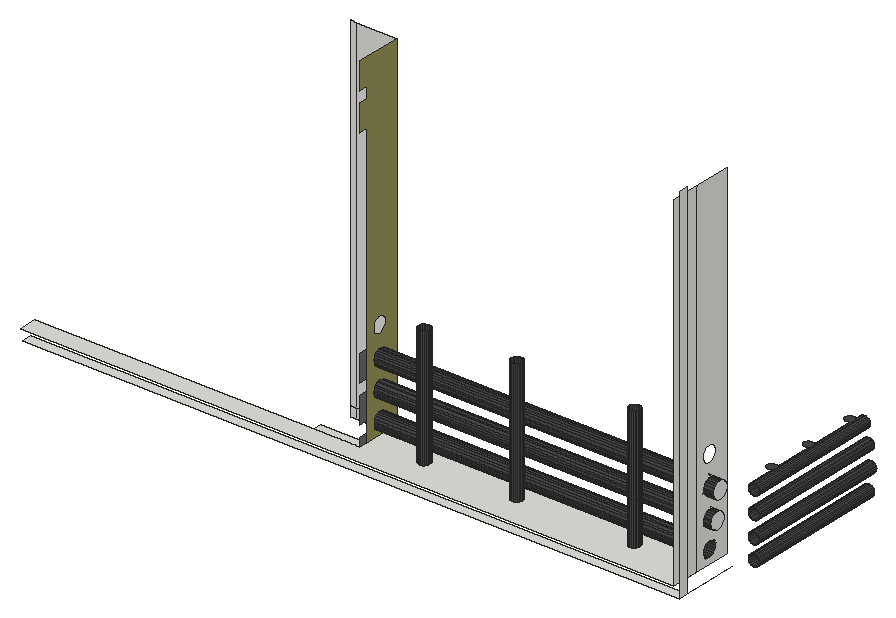
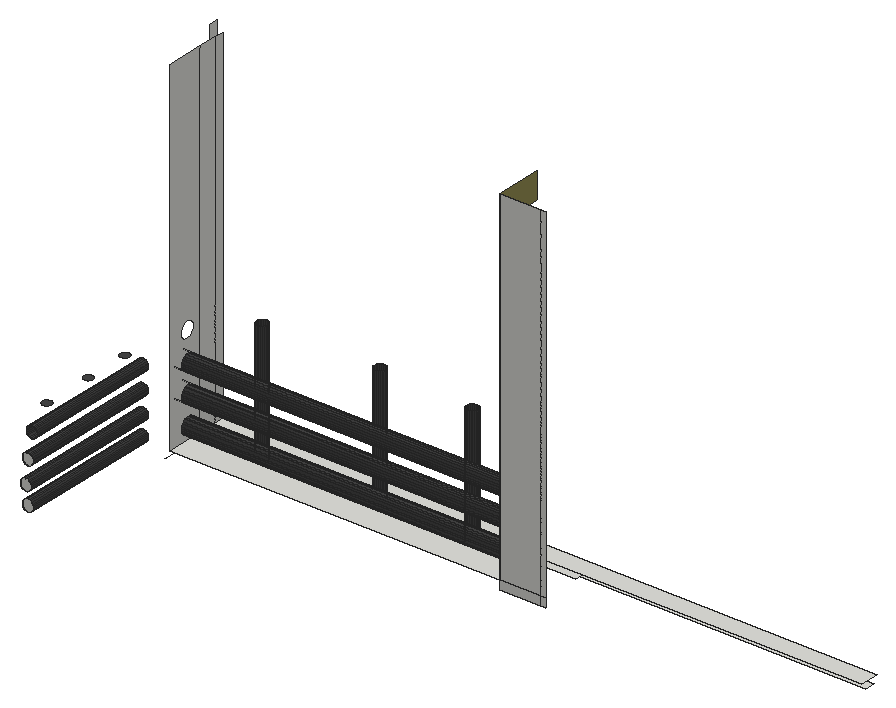
# SketchUp Ruby script. Lengths in inches.
U = 1.inch
M = Sketchup.active_model
def pt(a) = Geom::Point3d.new(a.map { |v| v * U })
def face(e, loops, mat)
  f = e.add_face(loops[0].map { |a| pt(a) })
  loops[1..].each { |l| e.add_face(l.map { |a| pt(a) }).erase! }
  f.material = f.back_material = mat if mat
  f
end
# faces: each face lists its corners as indices into pts; further lists are holes
def faces(e, pts, list, mat = nil) = list.each { |f| face(e, (f[0].is_a?(Array) ? f : [f]).map { |l| l.map { |i| pts[i] } }, mat) }
# xy, xz, yz: faces in a plane at the given z, y or x. An outline is a flat list of corners, or four numbers for a rectangle; further outlines are holes
def ring(l) = l.size == 4 ? [[l[0], l[1]], [l[2], l[1]], [l[2], l[3]], [l[0], l[3]]] : l.each_slice(2).to_a
def flat(e, list, mat, &to3) = list.each { |f| face(e, (f[0].is_a?(Array) ? f : [f]).map { |l| ring(l).map { |u, v| to3.(u, v) } }, mat) }
def xy(e, z, list, mat = nil) = flat(e, list, mat) { |x, y| [x, y, z] }
def xz(e, y, list, mat = nil) = flat(e, list, mat) { |x, z| [x, y, z] }
def yz(e, x, list, mat = nil) = flat(e, list, mat) { |y, z| [x, y, z] }
def lines(e, pts, list) = list.each { |a, b| e.add_line(pt(pts[a]), pt(pts[b])) }
# prism: a flat outline (further loops are holes) pulled along v
def prism(e, loops, v, mat = nil)
  f = face(e, loops, mat); d = Geom::Vector3d.new(v.map { |x| x * U })
  f.pushpull(f.normal.samedirection?(d) ? d.length : -d.length)
end
def box(e, o, s, mat = nil) = prism(e, [[o, [o[0] + s[0], o[1], o[2]], [o[0] + s[0], o[1] + s[1], o[2]], [o[0], o[1] + s[1], o[2]]]], [0, 0, s[2]], mat)
def at(x, y, z, deg = 0) = Geom::Transformation.translation(pt([x, y, z])) * Geom::Transformation.rotation(ORIGIN, Z_AXIS, deg.degrees)
def axes(o, x, y, z) = Geom::Transformation.new([*x, 0, *y, 0, *z, 0, *pt(o).to_a, 1])
def part(name) = M.definitions.add(name)
# library, detail: a bought-in or finely detailed component or shape, given as its bounding box
def library(name, o, s) = part(name).tap { |d| box(d.entities, o, s) }
def detail(e, o, s) = box(e.add_group.entities, o, s)
def put(e, d, t, mat = nil) = e.add_instance(d, t).tap { |i| i.material = mat if mat }
def group(e, t, mat = nil) = e.add_group.tap { |g| g.transformation = t; g.material = mat if mat }.entities
root = M.entities
M.materials.add("[0057_DarkKhaki]").color = [150, 145, 85]
M.materials.add("[0134_DimGray]").color = [105, 105, 105]
M.materials.add("[0137_Black]").color = [71, 71, 71]
xy(root,244.84,[[286.99,1.0625,497.49,4.0625]])
xy(root,247.89,[[[286.17,1.0625,495.71,1.0625,495.71,22.0625,390.0625,22.0625,390.0625,7.0625,286.17,7.0625],[437.11,9.5,436.64,9.5625,436.2,9.74,435.83,10.03,435.54,10.41,435.36,10.84,435.29,11.3125,435.36,11.78,435.54,12.22,435.83,12.6,436.2,12.88,436.64,13.0625,437.11,13.125,437.58,13.0625,438.01,12.88,438.39,12.6,438.68,12.22,438.86,11.78,438.92,11.3125,438.86,10.84,438.68,10.41,438.39,10.03,438.01,9.74,437.58,9.5625],[407.42,9.5,406.95,9.5625,406.51,9.74,406.14,10.03,405.85,10.41,405.67,10.84,405.61,11.3125,405.67,11.78,405.85,12.22,406.14,12.6,406.51,12.88,406.95,13.0625,407.42,13.125,407.89,13.0625,408.33,12.88,408.7,12.6,408.99,12.22,409.17,11.78,409.23,11.3125,409.17,10.84,408.99,10.41,408.7,10.03,408.33,9.74,407.89,9.5625],[474.86,9.5,474.39,9.5625,473.95,9.74,473.58,10.03,473.29,10.41,473.11,10.84,473.04,11.3125,473.11,11.78,473.29,12.22,473.58,12.6,473.95,12.88,474.39,13.0625,474.86,13.125,475.33,13.0625,475.76,12.88,476.14,12.6,476.43,12.22,476.61,11.78,476.67,11.3125,476.61,10.84,476.43,10.41,476.14,10.03,475.76,9.74,475.33,9.5625]],[375.29,7.0625,390.0625,10.0625]])
xy(root,274.04,[[505.89,26.06,506.26,26.11,506.6,26.25,506.9,26.48,507.13,26.78,507.27,27.125,507.32,27.5,507.27,27.87,507.13,28.22,506.9,28.51,506.6,28.74,506.26,28.89,505.89,28.93,505.51,28.89,505.17,28.74,504.87,28.51,504.64,28.22,504.5,27.87,504.45,27.5,504.5,27.125,504.64,26.78,504.87,26.48,505.17,26.25,505.51,26.11],[505.89,40.75,506.26,40.8,506.6,40.9375,506.9,41.17,507.13,41.47,507.27,41.8125,507.32,42.18,507.27,42.56,507.13,42.9,506.9,43.2,506.6,43.43,506.26,43.57,505.89,43.62,505.51,43.57,505.17,43.43,504.87,43.2,504.64,42.9,504.5,42.56,504.45,42.18,504.5,41.8125,504.64,41.47,504.87,41.17,505.17,40.9375,505.51,40.8],[505.89,57.31,506.26,57.36,506.6,57.5,506.9,57.73,507.13,58.03,507.27,58.375,507.32,58.75,507.27,59.12,507.13,59.47,506.9,59.76,506.6,59.99,506.26,60.14,505.89,60.18,505.51,60.14,505.17,59.99,504.87,59.76,504.64,59.47,504.5,59.12,504.45,58.75,504.5,58.375,504.64,58.03,504.87,57.73,505.17,57.5,505.51,57.36]],"[0137_Black]")
xz(root,22.0625,[[375.29,244.84,376.99,247.89],[376.99,244.84,390.0625,247.89],[375.29,247.89,376.99,358.6875],[376.99,247.89,390.0625,358.6875]])
xz(root,67.875,[[504.58,247.21,504.11,247.27,503.67,247.45,503.3,247.74,503.01,248.11,502.83,248.55,502.77,249.02,502.83,249.49,503.01,249.93,503.3,250.3,503.67,250.59,504.11,250.77,504.58,250.83,505.05,250.77,505.49,250.59,505.86,250.3,506.15,249.93,506.33,249.49,506.39,249.02,506.33,248.55,506.15,248.11,505.86,247.74,505.49,247.45,505.05,247.27],[504.58,260.58,504.11,260.64,503.67,260.83,503.3,261.11,503.01,261.49,502.83,261.93,502.77,262.39,502.83,262.86,503.01,263.3,503.3,263.68,503.67,263.96,504.11,264.15,504.58,264.21,505.05,264.15,505.49,263.96,505.86,263.68,506.15,263.3,506.33,262.86,506.39,262.39,506.33,261.93,506.15,261.49,505.86,261.11,505.49,260.83,505.05,260.64]])
xz(root,68.75,[[504.58,253.58,504.11,253.64,503.67,253.83,503.3,254.11,503.01,254.49,502.83,254.93,502.77,255.39,502.83,255.86,503.01,256.3,503.3,256.68,503.67,256.96,504.11,257.15,504.58,257.21,505.05,257.15,505.49,256.96,505.86,256.68,506.15,256.3,506.33,255.86,506.39,255.39,506.33,254.93,506.15,254.49,505.86,254.11,505.49,253.83,505.05,253.64]])
yz(root,390.0625,[[[10.0625,247.89,22.0625,247.89,22.0625,358.6875,7.0625,358.6875,7.0625,350.27,10.0625,350.27,10.0625,346.6875,7.0625,346.6875,7.0625,338.27,10.0625,338.27],[15.21,258.72,14.55,258.81,13.93,259.0625,13.4,259.47,12.99,260,12.73,260.62,12.65,261.28,12.73,261.95,12.99,262.5625,13.4,263.09,13.93,263.5,14.55,263.76,15.21,263.84,15.87,263.76,16.49,263.5,17.02,263.09,17.43,262.5625,17.68,261.95,17.77,261.28,17.68,260.62,17.43,260,17.02,259.47,16.49,259.0625,15.87,258.81],[15.21,267.84,14.55,267.93,13.93,268.1875,13.4,268.6,12.99,269.125,12.73,269.74,12.65,270.41,12.73,271.07,12.99,271.6875,13.4,272.22,13.93,272.625,14.55,272.88,15.21,272.97,15.87,272.88,16.49,272.625,17.02,272.22,17.43,271.6875,17.68,271.07,17.77,270.41,17.68,269.74,17.43,269.125,17.02,268.6,16.49,268.1875,15.87,267.93],[15.21,276.97,14.55,277.06,13.93,277.3125,13.4,277.72,12.99,278.25,12.73,278.87,12.65,279.53,12.73,280.2,12.99,280.8125,13.4,281.34,13.93,281.75,14.55,282.01,15.21,282.09,15.87,282.01,16.49,281.75,17.02,281.34,17.43,280.8125,17.68,280.2,17.77,279.53,17.68,278.87,17.43,278.25,17.02,277.72,16.49,277.3125,15.87,277.06],[15.21,249.59,14.55,249.68,13.93,249.9375,13.4,250.35,12.99,250.875,12.73,251.49,12.65,252.16,12.73,252.82,12.99,253.4375,13.4,253.97,13.93,254.375,14.55,254.63,15.21,254.72,15.87,254.63,16.49,254.375,17.02,253.97,17.43,253.4375,17.68,252.82,17.77,252.16,17.68,251.49,17.43,250.875,17.02,250.35,16.49,249.9375,15.87,249.68]]],"[0057_DarkKhaki]")
yz(root,390.0625,[[7.0625,247.89,10.0625,250.6875],[7.0625,254.27,10.0625,262.6875],[7.0625,266.27,10.0625,274.6875]],"[0134_DimGray]")
yz(root,495.71,[[1.0625,247.89,4.0625,358.6875],[4.0625,247.89,10.0625,358.6875],[[10.0625,247.89,22.0625,358.6875],[15.21,276.97,15.87,277.06,16.49,277.3125,17.02,277.72,17.43,278.25,17.68,278.87,17.77,279.53,17.68,280.2,17.43,280.8125,17.02,281.34,16.49,281.75,15.87,282.01,15.21,282.09,14.55,282.01,13.93,281.75,13.4,281.34,12.99,280.8125,12.73,280.2,12.65,279.53,12.73,278.87,12.99,278.25,13.4,277.72,13.93,277.3125,14.55,277.06],[15.21,249.59,15.87,249.68,16.49,249.9375,17.02,250.35,17.43,250.875,17.68,251.49,17.77,252.16,17.68,252.82,17.43,253.4375,17.02,253.97,16.49,254.375,15.87,254.63,15.21,254.72,14.55,254.63,13.93,254.375,13.4,253.97,12.99,253.4375,12.73,252.82,12.65,252.16,12.73,251.49,12.99,250.875,13.4,250.35,13.93,249.9375,14.55,249.68]]])
yz(root,497.49,[[1.0625,244.84,4.0625,361.64]])
yz(root,498.375,[[15.21,258.72,15.87,258.81,16.49,259.0625,17.02,259.47,17.43,260,17.68,260.62,17.77,261.28,17.68,261.95,17.43,262.5625,17.02,263.09,16.49,263.5,15.87,263.76,15.21,263.84,14.55,263.76,13.93,263.5,13.4,263.09,12.99,262.5625,12.73,261.95,12.65,261.28,12.73,260.62,12.99,260,13.4,259.47,13.93,259.0625,14.55,258.81]])
yz(root,499.25,[[15.21,267.84,15.87,267.93,16.49,268.1875,17.02,268.6,17.43,269.125,17.68,269.74,17.77,270.41,17.68,271.07,17.43,271.6875,17.02,272.22,16.49,272.625,15.87,272.88,15.21,272.97,14.55,272.88,13.93,272.625,13.4,272.22,12.99,271.6875,12.73,271.07,12.65,270.41,12.73,269.74,12.99,269.125,13.4,268.6,13.93,268.1875,14.55,267.93]])
p = [[504.58,22.0625,247.21],[504.11,22.0625,247.27],[504.11,67.875,247.27],[504.58,67.875,247.21],[505.05,22.0625,247.27],[505.05,67.875,247.27],
  [503.67,22.0625,247.45],[503.67,67.875,247.45],[505.49,22.0625,247.45],[505.49,67.875,247.45],[503.3,22.0625,247.74],[503.3,67.875,247.74],
  [505.86,22.0625,247.74],[505.86,67.875,247.74],[503.01,22.0625,248.11],[503.01,67.875,248.11],[506.15,22.0625,248.11],[506.15,67.875,248.11],
  [406.95,9.5625,247.89],[407.42,9.5,247.89],[407.42,9.5,286.45],[406.95,9.5625,286.45],[407.89,9.5625,247.89],[407.89,9.5625,286.45],
  [436.64,9.5625,247.89],[437.11,9.5,247.89],[437.11,9.5,287.52],[436.64,9.5625,287.52],[437.58,9.5625,247.89],[437.58,9.5625,287.52],
  [474.39,9.5625,247.89],[474.86,9.5,247.89],[474.86,9.5,287.08],[474.39,9.5625,287.08],[475.33,9.5625,247.89],[475.33,9.5625,287.08],
  [406.51,9.74,247.89],[406.51,9.74,286.45],[408.33,9.74,247.89],[408.33,9.74,286.45],[436.2,9.74,247.89],[436.2,9.74,287.52],
  [438.01,9.74,247.89],[438.01,9.74,287.52],[473.95,9.74,247.89],[473.95,9.74,287.08],[475.76,9.74,247.89],[475.76,9.74,287.08],
  [406.14,10.03,247.89],[406.14,10.03,286.45],[408.7,10.03,247.89],[408.7,10.03,286.45],[435.83,10.03,247.89],[435.83,10.03,287.52],
  [438.39,10.03,247.89],[438.39,10.03,287.52],[473.58,10.03,247.89],[473.58,10.03,287.08],[476.14,10.03,247.89],[476.14,10.03,287.08],
  [405.85,10.41,247.89],[405.85,10.41,286.45],[408.99,10.41,247.89],[408.99,10.41,286.45],[435.54,10.41,247.89],[435.54,10.41,287.52],
  [438.68,10.41,247.89],[438.68,10.41,287.52],[473.29,10.41,247.89],[473.29,10.41,287.08],[476.43,10.41,247.89],[476.43,10.41,287.08],
  [405.67,10.84,247.89],[405.67,10.84,286.45],[409.17,10.84,247.89],[409.17,10.84,286.45],[435.36,10.84,247.89],[435.36,10.84,287.52],
  [438.86,10.84,247.89],[438.86,10.84,287.52],[473.11,10.84,247.89],[473.11,10.84,287.08],[476.61,10.84,247.89],[476.61,10.84,287.08],
  [405.61,11.3125,247.89],[405.61,11.3125,286.45],[409.23,11.3125,247.89],[409.23,11.3125,286.45],[435.29,11.3125,247.89],[435.29,11.3125,287.52],
  [438.92,11.3125,247.89],[438.92,11.3125,287.52],[473.04,11.3125,247.89],[473.04,11.3125,287.08],[476.67,11.3125,247.89],[476.67,11.3125,287.08],
  [405.67,11.78,247.89],[405.67,11.78,286.45],[409.17,11.78,247.89],[409.17,11.78,286.45],[435.36,11.78,247.89],[435.36,11.78,287.52],
  [438.86,11.78,247.89],[438.86,11.78,287.52],[473.11,11.78,247.89],[473.11,11.78,287.08],[476.61,11.78,247.89],[476.61,11.78,287.08],
  [405.85,12.22,247.89],[405.85,12.22,286.45],[408.99,12.22,247.89],[408.99,12.22,286.45],[435.54,12.22,247.89],[435.54,12.22,287.52],
  [438.68,12.22,247.89],[438.68,12.22,287.52],[473.29,12.22,247.89],[473.29,12.22,287.08],[476.43,12.22,247.89],[476.43,12.22,287.08],
  [406.14,12.6,247.89],[406.14,12.6,286.45],[408.7,12.6,247.89],[408.7,12.6,286.45],[435.83,12.6,247.89],[435.83,12.6,287.52],
  [438.39,12.6,247.89],[438.39,12.6,287.52],[473.58,12.6,247.89],[473.58,12.6,287.08],[476.14,12.6,247.89],[476.14,12.6,287.08],
  [406.51,12.88,247.89],[406.51,12.88,286.45],[408.33,12.88,247.89],[408.33,12.88,286.45],[436.2,12.88,247.89],[436.2,12.88,287.52],
  [438.01,12.88,247.89],[438.01,12.88,287.52],[473.95,12.88,247.89],[473.95,12.88,287.08],[475.76,12.88,247.89],[475.76,12.88,287.08],
  [406.95,13.0625,247.89],[406.95,13.0625,286.45],[407.89,13.0625,247.89],[407.89,13.0625,286.45],[436.64,13.0625,247.89],[436.64,13.0625,287.52],
  [437.58,13.0625,247.89],[437.58,13.0625,287.52],[474.39,13.0625,247.89],[474.39,13.0625,287.08],[475.33,13.0625,247.89],[475.33,13.0625,287.08],
  [407.42,13.125,247.89],[407.42,13.125,286.45],[437.11,13.125,247.89],[437.11,13.125,287.52],[474.86,13.125,247.89],[474.86,13.125,287.08],
  [502.83,22.0625,248.55],[502.83,67.875,248.55],[506.33,22.0625,248.55],[506.33,67.875,248.55],[502.77,22.0625,249.02],[502.77,67.875,249.02],
  [506.39,22.0625,249.02],[506.39,67.875,249.02],[502.83,22.0625,249.49],[502.83,67.875,249.49],[506.33,22.0625,249.49],[506.33,67.875,249.49],
  [503.01,22.0625,249.93],[503.01,67.875,249.93],[506.15,22.0625,249.93],[506.15,67.875,249.93],[390.0625,14.55,249.68],[390.0625,15.21,249.59],
  [495.71,15.21,249.59],[495.71,14.55,249.68],[390.0625,15.87,249.68],[495.71,15.87,249.68],[390.0625,13.93,249.9375],[495.71,13.93,249.9375],
  [390.0625,16.49,249.9375],[495.71,16.49,249.9375],[390.0625,13.4,250.35],[495.71,13.4,250.35],[390.0625,17.02,250.35],[495.71,17.02,250.35],
  [503.3,22.0625,250.3],[503.3,67.875,250.3],[505.86,22.0625,250.3],[505.86,67.875,250.3],[390.0625,12.99,250.875],[495.71,12.99,250.875],
  [390.0625,17.43,250.875],[495.71,17.43,250.875],[503.67,22.0625,250.59],[503.67,67.875,250.59],[505.49,22.0625,250.59],[505.49,67.875,250.59],
  [504.11,22.0625,250.77],[504.11,67.875,250.77],[505.05,22.0625,250.77],[505.05,67.875,250.77],[504.58,22.0625,250.83],[504.58,67.875,250.83],
  [390.0625,12.73,251.49],[495.71,12.73,251.49],[390.0625,17.68,251.49],[495.71,17.68,251.49],[390.0625,12.65,252.16],[495.71,12.65,252.16],
  [390.0625,17.77,252.16],[495.71,17.77,252.16],[390.0625,12.73,252.82],[495.71,12.73,252.82],[390.0625,17.68,252.82],[495.71,17.68,252.82],
  [390.0625,12.99,253.4375],[495.71,12.99,253.4375],[390.0625,17.43,253.4375],[495.71,17.43,253.4375],[390.0625,13.4,253.97],[495.71,13.4,253.97],
  [390.0625,17.02,253.97],[495.71,17.02,253.97],[504.11,22.0625,253.64],[503.67,22.0625,253.83],[503.67,68.75,253.83],[504.11,68.75,253.64],
  [504.58,22.0625,253.58],[504.58,68.75,253.58],[505.05,22.0625,253.64],[505.05,68.75,253.64],[505.49,22.0625,253.83],[505.49,68.75,253.83],
  [503.3,22.0625,254.11],[503.3,68.75,254.11],[505.86,22.0625,254.11],[505.86,68.75,254.11],[390.0625,13.93,254.375],[495.71,13.93,254.375],
  [390.0625,16.49,254.375],[495.71,16.49,254.375],[503.01,22.0625,254.49],[503.01,68.75,254.49],[506.15,22.0625,254.49],[506.15,68.75,254.49],
  [390.0625,14.55,254.63],[495.71,14.55,254.63],[390.0625,15.87,254.63],[495.71,15.87,254.63],[502.83,22.0625,254.93],[502.83,68.75,254.93],
  [506.33,22.0625,254.93],[506.33,68.75,254.93],[390.0625,15.21,254.72],[495.71,15.21,254.72],[502.77,22.0625,255.39],[502.77,68.75,255.39],
  [506.39,22.0625,255.39],[506.39,68.75,255.39],[502.83,22.0625,255.86],[502.83,68.75,255.86],[506.33,22.0625,255.86],[506.33,68.75,255.86],
  [503.01,22.0625,256.3],[503.01,68.75,256.3],[506.15,22.0625,256.3],[506.15,68.75,256.3],[503.3,22.0625,256.68],[503.3,68.75,256.68],
  [505.86,22.0625,256.68],[505.86,68.75,256.68],[503.67,22.0625,256.96],[503.67,68.75,256.96],[505.49,22.0625,256.96],[505.49,68.75,256.96],
  [504.11,22.0625,257.15],[504.11,68.75,257.15],[505.05,22.0625,257.15],[505.05,68.75,257.15],[504.58,22.0625,257.21],[504.58,68.75,257.21],
  [390.0625,14.55,258.81],[390.0625,15.21,258.72],[498.375,15.21,258.72],[498.375,14.55,258.81],[390.0625,15.87,258.81],[498.375,15.87,258.81],
  [390.0625,13.93,259.0625],[498.375,13.93,259.0625],[390.0625,16.49,259.0625],[498.375,16.49,259.0625],[390.0625,13.4,259.47],[498.375,13.4,259.47],
  [390.0625,17.02,259.47],[498.375,17.02,259.47],[390.0625,12.99,260],[498.375,12.99,260],[390.0625,17.43,260],[498.375,17.43,260],
  [390.0625,12.73,260.62],[498.375,12.73,260.62],[390.0625,17.68,260.62],[498.375,17.68,260.62],[390.0625,12.65,261.28],[498.375,12.65,261.28],
  [390.0625,17.77,261.28],[498.375,17.77,261.28],[504.11,22.0625,260.64],[503.67,22.0625,260.83],[503.67,67.875,260.83],[504.11,67.875,260.64],
  [504.58,22.0625,260.58],[504.58,67.875,260.58],[505.05,22.0625,260.64],[505.05,67.875,260.64],[505.49,22.0625,260.83],[505.49,67.875,260.83],
  [503.3,22.0625,261.11],[503.3,67.875,261.11],[505.86,22.0625,261.11],[505.86,67.875,261.11],[503.01,22.0625,261.49],[503.01,67.875,261.49],
  [506.15,22.0625,261.49],[506.15,67.875,261.49],[390.0625,12.73,261.95],[498.375,12.73,261.95],[390.0625,17.68,261.95],[498.375,17.68,261.95],
  [502.83,22.0625,261.93],[502.83,67.875,261.93],[506.33,22.0625,261.93],[506.33,67.875,261.93],[390.0625,12.99,262.5625],[498.375,12.99,262.5625],
  [390.0625,17.43,262.5625],[498.375,17.43,262.5625],[502.77,22.0625,262.39],[502.77,67.875,262.39],[506.39,22.0625,262.39],[506.39,67.875,262.39],
  [502.83,22.0625,262.86],[502.83,67.875,262.86],[506.33,22.0625,262.86],[506.33,67.875,262.86],[390.0625,13.4,263.09],[498.375,13.4,263.09],
  [390.0625,17.02,263.09],[498.375,17.02,263.09],[503.01,22.0625,263.3],[503.01,67.875,263.3],[506.15,22.0625,263.3],[506.15,67.875,263.3],
  [390.0625,13.93,263.5],[498.375,13.93,263.5],[390.0625,16.49,263.5],[498.375,16.49,263.5],[503.3,22.0625,263.68],[503.3,67.875,263.68],
  [505.86,22.0625,263.68],[505.86,67.875,263.68],[390.0625,14.55,263.76],[498.375,14.55,263.76],[390.0625,15.87,263.76],[498.375,15.87,263.76],
  [503.67,22.0625,263.96],[503.67,67.875,263.96],[505.49,22.0625,263.96],[505.49,67.875,263.96],[390.0625,15.21,263.84],[498.375,15.21,263.84],
  [504.11,22.0625,264.15],[504.11,67.875,264.15],[505.05,22.0625,264.15],[505.05,67.875,264.15],[504.58,22.0625,264.21],[504.58,67.875,264.21],
  [504.11,22.0625,267.64],[503.67,22.0625,267.83],[503.67,66.25,267.83],[504.11,66.25,267.64],[504.58,22.0625,267.58],[504.58,66.25,267.58],
  [505.05,22.0625,267.64],[505.05,66.25,267.64],[505.49,22.0625,267.83],[505.49,66.25,267.83],[390.0625,14.55,267.93],[390.0625,15.21,267.84],
  [499.25,15.21,267.84],[499.25,14.55,267.93],[390.0625,15.87,267.93],[499.25,15.87,267.93],[503.3,22.0625,268.11],[503.3,66.25,268.11],
  [505.86,22.0625,268.11],[505.86,66.25,268.11],[390.0625,13.93,268.1875],[499.25,13.93,268.1875],[390.0625,16.49,268.1875],[499.25,16.49,268.1875],
  [503.01,22.0625,268.49],[503.01,66.25,268.49],[506.15,22.0625,268.49],[506.15,66.25,268.49],[390.0625,13.4,268.6],[499.25,13.4,268.6],
  [390.0625,17.02,268.6],[499.25,17.02,268.6],[502.83,22.0625,268.93],[502.83,66.25,268.93],[506.33,22.0625,268.93],[506.33,66.25,268.93],
  [390.0625,12.99,269.125],[499.25,12.99,269.125],[390.0625,17.43,269.125],[499.25,17.43,269.125],[502.77,22.0625,269.39],[502.77,66.25,269.39],
  [506.39,22.0625,269.39],[506.39,66.25,269.39],[390.0625,12.73,269.74],[499.25,12.73,269.74],[390.0625,17.68,269.74],[499.25,17.68,269.74],
  [502.83,22.0625,269.86],[502.83,66.25,269.86],[506.33,22.0625,269.86],[506.33,66.25,269.86],[390.0625,12.65,270.41],[499.25,12.65,270.41],
  [390.0625,17.77,270.41],[499.25,17.77,270.41],[503.01,22.0625,270.3],[503.01,66.25,270.3],[506.15,22.0625,270.3],[506.15,66.25,270.3],
  [503.3,22.0625,270.68],[503.3,66.25,270.68],[505.86,22.0625,270.68],[505.86,66.25,270.68],[390.0625,12.73,271.07],[499.25,12.73,271.07],
  [390.0625,17.68,271.07],[499.25,17.68,271.07],[503.67,22.0625,270.96],[503.67,66.25,270.96],[505.49,22.0625,270.96],[505.49,66.25,270.96],
  [504.11,22.0625,271.15],[504.11,66.25,271.15],[505.05,22.0625,271.15],[505.05,66.25,271.15],[390.0625,12.99,271.6875],[499.25,12.99,271.6875],
  [390.0625,17.43,271.6875],[499.25,17.43,271.6875],[504.58,22.0625,271.21],[504.58,66.25,271.21],[390.0625,13.4,272.22],[499.25,13.4,272.22],
  [390.0625,17.02,272.22],[499.25,17.02,272.22],[390.0625,13.93,272.625],[499.25,13.93,272.625],[390.0625,16.49,272.625],[499.25,16.49,272.625],
  [390.0625,14.55,272.88],[499.25,14.55,272.88],[390.0625,15.87,272.88],[499.25,15.87,272.88],[390.0625,15.21,272.97],[499.25,15.21,272.97],
  [497.49,4.0625,244.84],[497.49,22.0625,244.84]]
faces(root,p,[[0,1,2,3],[4,0,3,5],[1,6,7,2],[8,4,5,9],[6,10,11,7],[12,8,9,13],[10,14,15,11],[16,12,13,17],
  [18,19,20,21],[19,22,23,20],[24,25,26,27],[25,28,29,26],[30,31,32,33],[31,34,35,32],[36,18,21,37],[22,38,39,23],
  [40,24,27,41],[28,42,43,29],[44,30,33,45],[34,46,47,35],[48,36,37,49],[38,50,51,39],[52,40,41,53],[42,54,55,43],
  [56,44,45,57],[46,58,59,47],[60,48,49,61],[50,62,63,51],[64,52,53,65],[54,66,67,55],[68,56,57,69],[58,70,71,59],
  [72,60,61,73],[62,74,75,63],[76,64,65,77],[66,78,79,67],[80,68,69,81],[70,82,83,71],[84,72,73,85],[74,86,87,75],
  [88,76,77,89],[78,90,91,79],[92,80,81,93],[82,94,95,83],[96,84,85,97],[86,98,99,87],[100,88,89,101],[90,102,103,91],
  [104,92,93,105],[94,106,107,95],[108,96,97,109],[98,110,111,99],[112,100,101,113],[102,114,115,103],[116,104,105,117],[106,118,119,107],
  [120,108,109,121],[110,122,123,111],[124,112,113,125],[114,126,127,115],[128,116,117,129],[118,130,131,119],[132,120,121,133],[122,134,135,123],
  [136,124,125,137],[126,138,139,127],[140,128,129,141],[130,142,143,131],[144,132,133,145],[134,146,147,135],[148,136,137,149],[138,150,151,139],
  [152,140,141,153],[142,154,155,143],[156,144,145,157],[146,156,157,147],[158,148,149,159],[150,158,159,151],[160,152,153,161],[154,160,161,155],
  [14,162,163,15],[164,16,17,165],[162,166,167,163],[168,164,165,169],[166,170,171,167],[172,168,169,173],[170,174,175,171],[176,172,173,177],
  [178,179,180,181],[179,182,183,180],[184,178,181,185],[182,186,187,183],[188,184,185,189],[186,190,191,187],[174,192,193,175],[194,176,177,195],
  [196,188,189,197],[190,198,199,191],[192,200,201,193],[202,194,195,203],[200,204,205,201],[206,202,203,207],[204,208,209,205],[208,206,207,209],
  [210,196,197,211],[198,212,213,199],[214,210,211,215],[212,216,217,213],[218,214,215,219],[216,220,221,217],[222,218,219,223],[220,224,225,221],
  [226,222,223,227],[224,228,229,225],[230,231,232,233],[234,230,233,235],[236,234,235,237],[238,236,237,239],[231,240,241,232],[242,238,239,243],
  [244,226,227,245],[228,246,247,229],[240,248,249,241],[250,242,243,251],[252,244,245,253],[246,254,255,247],[248,256,257,249],[258,250,251,259],
  [260,252,253,261],[254,260,261,255],[256,262,263,257],[264,258,259,265],[262,266,267,263],[268,264,265,269],[266,270,271,267],[272,268,269,273],
  [270,274,275,271],[276,272,273,277],[274,278,279,275],[280,276,277,281],[278,282,283,279],[284,280,281,285],[282,286,287,283],[286,284,285,287],
  [288,289,290,291],[289,292,293,290],[294,288,291,295],[292,296,297,293],[298,294,295,299],[296,300,301,297],[302,298,299,303],[300,304,305,301],
  [306,302,303,307],[304,308,309,305],[310,306,307,311],[308,312,313,309],[314,315,316,317],[318,314,317,319],[320,318,319,321],[322,320,321,323],
  [315,324,325,316],[326,322,323,327],[324,328,329,325],[330,326,327,331],[332,310,311,333],[312,334,335,313],[328,336,337,329],[338,330,331,339],
  [340,332,333,341],[334,342,343,335],[336,344,345,337],[346,338,339,347],[344,348,349,345],[350,346,347,351],[352,340,341,353],[342,354,355,343],
  [348,356,357,349],[358,350,351,359],[360,352,353,361],[354,362,363,355],[356,364,365,357],[366,358,359,367],[368,360,361,369],[362,370,371,363],
  [364,372,373,365],[374,366,367,375],[376,368,369,377],[370,376,377,371],[372,378,379,373],[380,374,375,381],[378,382,383,379],[382,380,381,383],
  [384,385,386,387],[388,384,387,389],[390,388,389,391],[392,390,391,393],[394,395,396,397],[395,398,399,396],[385,400,401,386],[402,392,393,403],
  [404,394,397,405],[398,406,407,399],[400,408,409,401],[410,402,403,411],[412,404,405,413],[406,414,415,407],[408,416,417,409],[418,410,411,419],
  [420,412,413,421],[414,422,423,415],[416,424,425,417],[426,418,419,427],[428,420,421,429],[422,430,431,423],[424,432,433,425],[434,426,427,435],
  [436,428,429,437],[430,438,439,431],[432,440,441,433],[442,434,435,443],[440,444,445,441],[446,442,443,447],[448,436,437,449],[438,450,451,439],
  [444,452,453,445],[454,446,447,455],[452,456,457,453],[458,454,455,459],[460,448,449,461],[450,462,463,451],[456,464,465,457],[464,458,459,465],
  [466,460,461,467],[462,468,469,463],[470,466,467,471],[468,472,473,469],[474,470,471,475],[472,476,477,473],[478,474,475,479],[476,478,479,477]],"[0137_Black]")
lines(root,p,[[480,481]])
